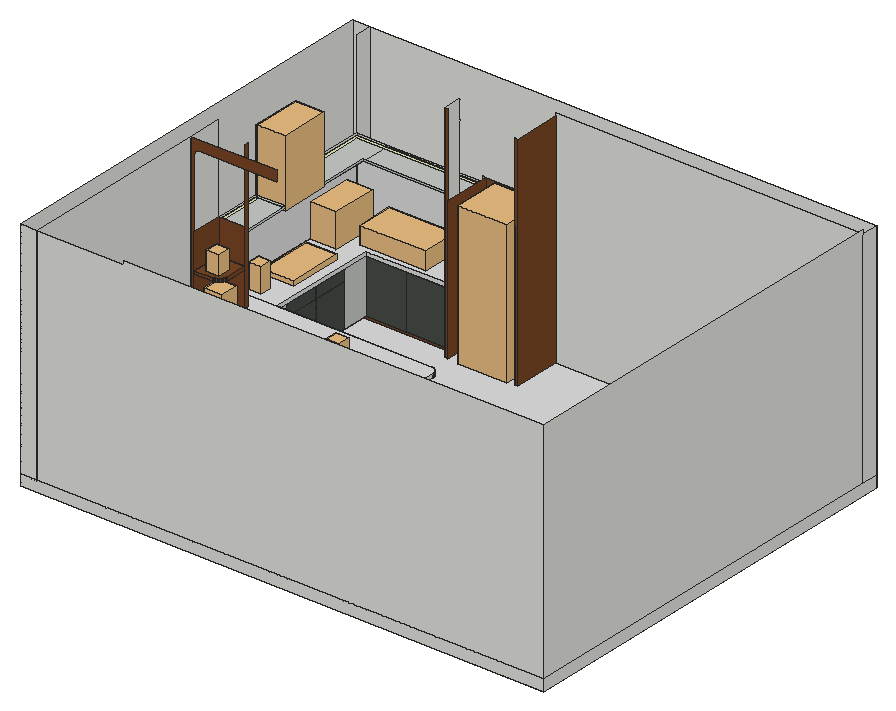
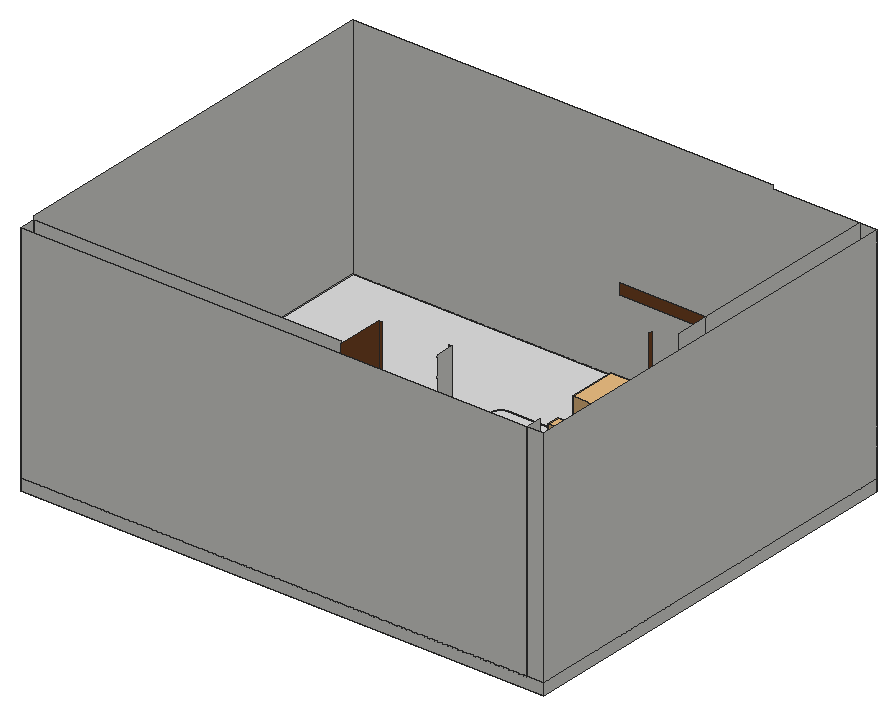
# SketchUp Ruby script. Lengths in inches.
U = 1.inch
M = Sketchup.active_model
def pt(a) = Geom::Point3d.new(a.map { |v| v * U })
def face(e, loops, mat)
  f = e.add_face(loops[0].map { |a| pt(a) })
  loops[1..].each { |l| e.add_face(l.map { |a| pt(a) }).erase! }
  f.material = f.back_material = mat if mat
  f
end
# faces: each face lists its corners as indices into pts; further lists are holes
def faces(e, pts, list, mat = nil) = list.each { |f| face(e, (f[0].is_a?(Array) ? f : [f]).map { |l| l.map { |i| pts[i] } }, mat) }
# xy, xz, yz: faces in a plane at the given z, y or x. An outline is a flat list of corners, or four numbers for a rectangle; further outlines are holes
def ring(l) = l.size == 4 ? [[l[0], l[1]], [l[2], l[1]], [l[2], l[3]], [l[0], l[3]]] : l.each_slice(2).to_a
def flat(e, list, mat, &to3) = list.each { |f| face(e, (f[0].is_a?(Array) ? f : [f]).map { |l| ring(l).map { |u, v| to3.(u, v) } }, mat) }
def xy(e, z, list, mat = nil) = flat(e, list, mat) { |x, y| [x, y, z] }
def xz(e, y, list, mat = nil) = flat(e, list, mat) { |x, z| [x, y, z] }
def yz(e, x, list, mat = nil) = flat(e, list, mat) { |y, z| [x, y, z] }
def lines(e, pts, list) = list.each { |a, b| e.add_line(pt(pts[a]), pt(pts[b])) }
# prism: a flat outline (further loops are holes) pulled along v
def prism(e, loops, v, mat = nil)
  f = face(e, loops, mat); d = Geom::Vector3d.new(v.map { |x| x * U })
  f.pushpull(f.normal.samedirection?(d) ? d.length : -d.length)
end
def box(e, o, s, mat = nil) = prism(e, [[o, [o[0] + s[0], o[1], o[2]], [o[0] + s[0], o[1] + s[1], o[2]], [o[0], o[1] + s[1], o[2]]]], [0, 0, s[2]], mat)
def at(x, y, z, deg = 0) = Geom::Transformation.translation(pt([x, y, z])) * Geom::Transformation.rotation(ORIGIN, Z_AXIS, deg.degrees)
def axes(o, x, y, z) = Geom::Transformation.new([*x, 0, *y, 0, *z, 0, *pt(o).to_a, 1])
def part(name) = M.definitions.add(name)
# library, detail: a bought-in or finely detailed component or shape, given as its bounding box
def library(name, o, s) = part(name).tap { |d| box(d.entities, o, s) }
def detail(e, o, s) = box(e.add_group.entities, o, s)
def put(e, d, t, mat = nil) = e.add_instance(d, t).tap { |i| i.material = mat if mat }
def group(e, t, mat = nil) = e.add_group.tap { |g| g.transformation = t; g.material = mat if mat }.entities
root = M.entities
M.materials.add("Emissive").color = [223, 228, 179]
M.materials.add("Generic").color = [71, 77, 71]
M.materials.add("Generic\#1").color = [198, 203, 199]
M.materials.add("Gold 10k").color = [251, 232, 180]
M.materials.add("Marble White SSS 100cm").color = [222, 222, 222]
M.materials.add("[Wood Veneer 01]").color = [120, 70, 37]
c1 = library("Refrigerator 300 009",[-13.27,-13.92,-0.16],[26.54,24.77,79.78])
c2 = library("Potted Plant 50-23",[-3.4,-3.5,0],[6.8,7,9.93])
c3 = library("Kitchen Sink 180 043",[-17.78,-9.92,-5.26],[35.55,19.84,14.38])
c4 = library("ACCESS \#103",[-1.07,0,-1.17],[14.88,24.44,20.18])
c5 = library("Utensils",[0,-0.54,-0.24],[6.34,6.28,13.37])
c6 = library("GasStove_Black",[0,0,0],[28.74,16.54,2.72])
c7 = library("Vase Lilies 26-19",[-4.61,-5.04,0],[9.42,9.94,10.95])
c8 = library("Tlon Light 1950 Ceiling 152 010",[-38.39,-38.39,-3.78],[76.78,76.78,3.41])
c9 = library("BERG+Spring+90",[0,0,0],[34.65,15.32,35.9])
xy(root,-6,[[0,0,280.625,223.125]])
xy(root,0,[[0,0,9,223.125],[9,0,10.8125,103.125],[9,103.125,10.8125,103.125,10.8125,107.125,33,107.125,33,123.125,29,123.125,29,194.125,33,194.125,33,214.125,9,214.125],[33,107.125,116,123.125],[33,107.125,116,123.125],
  [76.5,188.8125,78.25,188.8125,78.25,214.125,33,214.125,33,194.125,76.5,194.125],[76.5,188.8125,78.25,214.125],[114.125,188.8125,115.875,214.125],[114.125,188.8125,115.875,214.125],[33,194.125,76.5,214.125],
  [9,214.125,280.625,223.125]])
xy(root,0,[[10.8125,0,280.625,0,280.625,214.125,115.875,214.125,115.875,188.8125,114.125,188.8125,114.125,214.125,78.25,214.125,78.25,188.8125,76.5,188.8125,76.5,194.125,29,194.125,29,123.125,116,123.125,116,107.125,10.8125,107.125]],"Marble White SSS 100cm")
xy(root,4,[[10.8125,107.125,10.8125,120.99,9,120.99,9,214.125,76.5,214.125,76.5,194.125,29,194.125,29,123.125,116,123.125,116,107.125]])
xy(root,4,[[10.8125,106.18,10.8125,107.125,116,107.125,116,123.125,29,123.125,29,194.125,76.5,194.125,76.5,193.18,29.95,193.18,29.95,124.07,116.95,124.07,116.95,106.18]],"Emissive")
xy(root,4,[[10.8125,104.5625,10.8125,106.18,21.4375,106.18,21.4375,104.5625,18.3,104.5625,18.3,105.3125,17.9,105.3125,17.9,104.5625,14.75,104.5625,14.75,105.3125,14.35,105.3125,14.35,104.5625],[21.84,104.5625,24.98,106.18],[25.38,104.5625,28.52,106.18],[28.92,104.5625,32.0625,106.18],[99.36,104.5625,99.36,106.18,116.95,106.18,116.95,124.07,29.95,124.07,29.95,193.18,76.5,193.18,76.5,190.125,33,190.125,33,125.6875,117.27,125.6875,117.4375,125.68,117.6,125.64,117.76,125.59,117.92,125.51,118.06,125.42,118.18,125.31,118.29,125.18,118.39,125.04,118.46,124.89,118.52,124.73,118.53,124.6875,118.98,123.14,119.37,121.57,119.68,119.99,119.93,118.39,120.11,116.79,120.21,115.18,120.21,111.95,120.1,110.34,119.92,108.74,119.67,107.14,119.66,107.125,119.35,105.5625,118.48,105.5625,118.45,105.48,118.36,105.31,118.25,105.15,118.125,105,117.98,104.87,117.82,104.76,117.64,104.68,117.46,104.61,117.27,104.58,117.07,104.5625,117.07,105.3125,116.67,105.3125,116.67,104.5625,113.53,104.5625,113.53,105.3125,113.13,105.3125,113.13,104.5625,109.99,104.5625,109.99,105.3125,109.59,105.3125,109.59,104.5625,106.45,104.5625,106.45,105.3125,106.05,105.3125,106.05,104.5625,102.9,104.5625,102.9,105.3125,102.5,105.3125,102.5,104.5625],
  [32.46,104.5625,35.61,106.18],[36.01,104.5625,39.15,106.18],[39.55,104.5625,42.69,106.18],[43.09,104.5625,46.23,106.18],[46.63,104.5625,49.77,106.18],
  [50.17,104.5625,50.17,106.18,91.88,106.18,91.88,104.5625,88.74,104.5625,88.74,105.3125,88.34,105.3125,88.34,104.5625,85.19,104.5625,85.19,105.3125,84.79,105.3125,84.79,104.5625,81.65,104.5625,81.65,105.3125,81.25,105.3125,81.25,104.5625,78.51,104.5625,78.51,105.3125,78.11,105.3125,78.11,104.5625,74.97,104.5625,74.97,105.3125,74.57,105.3125,74.57,104.5625,71.43,104.5625,71.43,105.3125,71.03,105.3125,71.03,104.5625,67.88,104.5625,67.88,105.3125,67.48,105.3125,67.48,104.5625,64.34,104.5625,64.34,105.3125,63.94,105.3125,63.94,104.5625,60.8,104.5625,60.8,105.3125,60.4,105.3125,60.4,104.5625,57.26,104.5625,57.26,105.3125,56.86,105.3125,56.86,104.5625,53.72,104.5625,53.72,105.3125,53.32,105.3125,53.32,104.5625],[92.28,104.5625,95.42,106.18],[95.82,104.5625,98.96,106.18]],"[Wood Veneer 01]")
xy(root,5,[[112.375,105.5625,119.35,105.5625,119.66,107.125,119.67,107.14,119.92,108.74,120.1,110.34,120.21,111.95,120.21,115.18,120.11,116.79,119.93,118.39,119.68,119.99,119.37,121.57,118.98,123.14,118.53,124.6875,112.375,124.6875]],"[Wood Veneer 01]")
xy(root,13.49,[[112.375,105.5625,112.375,124.6875,118.53,124.6875,119.04,123.14,119.47,121.57,119.8,119.98,120.03,118.37,120.17,116.75,120.21,115.12,120.16,113.49,120.01,111.875,119.77,110.26,119.43,108.67,119,107.1,118.48,105.5625]],"[Wood Veneer 01]")
xy(root,14.08,[[112.375,105.5625,118.48,105.5625,119,107.1,119.43,108.67,119.77,110.26,120.01,111.875,120.16,113.49,120.21,115.12,120.17,116.75,120.03,118.37,119.8,119.98,119.47,121.57,119.04,123.14,118.53,124.6875,112.375,124.6875]],"[Wood Veneer 01]")
xy(root,22.24,[[112.375,105.5625,112.375,124.6875,118.53,124.6875,119.04,123.14,119.46,121.57,119.79,119.98,120.03,118.37,120.17,116.75,120.21,115.12,120.16,113.49,120.01,111.875,119.77,110.26,119.43,108.67,119,107.1,118.48,105.5625]],"[Wood Veneer 01]")
xy(root,22.83,[[112.375,105.5625,118.48,105.5625,119,107.1,119.43,108.67,119.77,110.26,120.01,111.875,120.16,113.49,120.21,115.12,120.17,116.75,120.03,118.37,119.79,119.98,119.46,121.57,119.04,123.14,118.53,124.6875,112.375,124.6875]],"[Wood Veneer 01]")
xy(root,32,[[112.375,105.5625,112.375,124.6875,118.53,124.6875,118.55,124.5625,118.5625,124.39,118.5625,106.05,118.55,105.86,118.51,105.67,118.48,105.5625]],"[Wood Veneer 01]")
xy(root,33,[[10.8125,104.5625,10.8125,120.99,9,120.99,9,214.125,76.5,214.125,76.5,190.125,33,190.125,33,125.6875,117.07,125.6875,117.07,105.3125,116.67,105.3125,116.67,104.5625,113.53,104.5625,113.53,105.3125,113.13,105.3125,113.13,104.5625,109.99,104.5625,109.99,105.3125,109.59,105.3125,109.59,104.5625,106.45,104.5625,106.45,105.3125,106.05,105.3125,106.05,104.5625,102.9,104.5625,102.9,105.3125,102.5,105.3125,102.5,104.5625,99.36,104.5625,99.36,106.18,98.96,106.18,98.96,104.5625,95.82,104.5625,95.82,106.18,95.42,106.18,95.42,104.5625,92.28,104.5625,92.28,106.18,91.88,106.18,91.88,104.5625,88.74,104.5625,88.74,105.3125,88.34,105.3125,88.34,104.5625,85.19,104.5625,85.19,105.3125,84.79,105.3125,84.79,104.5625,81.65,104.5625,81.65,105.3125,81.25,105.3125,81.25,104.5625,78.51,104.5625,78.51,105.3125,78.11,105.3125,78.11,104.5625,74.97,104.5625,74.97,105.3125,74.57,105.3125,74.57,104.5625,71.43,104.5625,71.43,105.3125,71.03,105.3125,71.03,104.5625,67.88,104.5625,67.88,105.3125,67.48,105.3125,67.48,104.5625,64.34,104.5625,64.34,105.3125,63.94,105.3125,63.94,104.5625,60.8,104.5625,60.8,105.3125,60.4,105.3125,60.4,104.5625,57.26,104.5625,57.26,105.3125,56.86,105.3125,56.86,104.5625,53.72,104.5625,53.72,105.3125,53.32,105.3125,53.32,104.5625,50.17,104.5625,50.17,106.18,49.77,106.18,49.77,104.5625,46.63,104.5625,46.63,106.18,46.23,106.18,46.23,104.5625,43.09,104.5625,43.09,106.18,42.69,106.18,42.69,104.5625,39.55,104.5625,39.55,106.18,39.15,106.18,39.15,104.5625,36.01,104.5625,36.01,106.18,35.61,106.18,35.61,104.5625,32.46,104.5625,32.46,106.18,32.0625,106.18,32.0625,104.5625,28.92,104.5625,28.92,106.18,28.52,106.18,28.52,104.5625,25.38,104.5625,25.38,106.18,24.98,106.18,24.98,104.5625,21.84,104.5625,21.84,106.18,21.4375,106.18,21.4375,104.5625,18.3,104.5625,18.3,105.3125,17.9,105.3125,17.9,104.5625,14.75,104.5625,14.75,105.3125,14.35,105.3125,14.35,104.5625],[117.07,104.5625,117.27,104.58,117.46,104.61,117.64,104.68,117.82,104.76,117.98,104.87,118.125,105,118.25,105.15,118.36,105.31,118.45,105.48,118.51,105.67,118.55,105.86,118.5625,106.05,118.5625,124.39,118.55,124.5625,118.52,124.73,118.46,124.89,118.39,125.04,118.29,125.18,118.18,125.31,118.06,125.42,117.92,125.51,117.76,125.59,117.6,125.64,117.4375,125.68,117.27,125.6875,117.07,125.6875]])
xy(root,33,[[10.8125,103.8125,10.8125,104.5625,14.35,104.5625,14.35,105.3125,14.75,105.3125,14.75,104.5625,17.9,104.5625,17.9,105.3125,18.3,105.3125,18.3,104.5625,21.4375,104.5625,21.4375,106.18,21.84,106.18,21.84,104.5625,24.98,104.5625,24.98,106.18,25.38,106.18,25.38,104.5625,28.52,104.5625,28.52,106.18,28.92,106.18,28.92,104.5625,32.0625,104.5625,32.0625,106.18,32.46,106.18,32.46,104.5625,35.61,104.5625,35.61,106.18,36.01,106.18,36.01,104.5625,39.15,104.5625,39.15,106.18,39.55,106.18,39.55,104.5625,42.69,104.5625,42.69,106.18,43.09,106.18,43.09,104.5625,46.23,104.5625,46.23,106.18,46.63,106.18,46.63,104.5625,49.77,104.5625,49.77,106.18,50.17,106.18,50.17,104.5625,53.32,104.5625,53.32,105.3125,53.72,105.3125,53.72,104.5625,56.86,104.5625,56.86,105.3125,57.26,105.3125,57.26,104.5625,60.4,104.5625,60.4,105.3125,60.8,105.3125,60.8,104.5625,63.94,104.5625,63.94,105.3125,64.34,105.3125,64.34,104.5625,67.48,104.5625,67.48,105.3125,67.88,105.3125,67.88,104.5625,71.03,104.5625,71.03,105.3125,71.43,105.3125,71.43,104.5625,74.57,104.5625,74.57,105.3125,74.97,105.3125,74.97,104.5625,78.11,104.5625,78.11,105.3125,78.51,105.3125,78.51,104.5625,81.25,104.5625,81.25,105.3125,81.65,105.3125,81.65,104.5625,84.79,104.5625,84.79,105.3125,85.19,105.3125,85.19,104.5625,88.34,104.5625,88.34,105.3125,88.74,105.3125,88.74,104.5625,91.88,104.5625,91.88,106.18,92.28,106.18,92.28,104.5625,95.42,104.5625,95.42,106.18,95.82,106.18,95.82,104.5625,98.96,104.5625,98.96,106.18,99.36,106.18,99.36,104.5625,102.5,104.5625,102.5,105.3125,102.9,105.3125,102.9,104.5625,106.05,104.5625,106.05,105.3125,106.45,105.3125,106.45,104.5625,109.59,104.5625,109.59,105.3125,109.99,105.3125,109.99,104.5625,113.13,104.5625,113.13,105.3125,113.53,105.3125,113.53,104.5625,116.67,104.5625,116.67,105.3125,117.07,105.3125,117.07,103.8125],[117.07,103.8125,117.07,104.5625,117.27,104.58,117.46,104.61,117.64,104.68,117.82,104.76,117.98,104.87,118.125,105,118.25,105.15,118.36,105.31,118.45,105.48,118.51,105.67,118.55,105.86,118.5625,106.05,118.5625,124.39,118.55,124.5625,118.52,124.73,118.46,124.89,118.39,125.04,118.29,125.18,118.18,125.31,118.06,125.42,117.92,125.51,117.76,125.59,117.6,125.64,117.4375,125.68,117.27,125.6875,117.07,125.6875,117.07,126.4375,119.125,126.4375,119.125,103.8125],[33,125.6875,117.07,126.4375]],"Emissive")
xy(root,34,[[120.76,103.125,120.8125,103.125,120.8125,103.21],[120.8125,103.21,120.99,103.48,121.27,104.03,121.46,104.62,121.58,105.22,121.625,105.83,121.625,124.4,121.58,125.02,121.46,125.62,121.27,126.21,120.99,126.76,120.8125,127.03],[10.8125,103.8125,10.8125,120.99,9,120.99,9,214.125,76.5,214.125,76.5,190.125,33,190.125,33,126.4375,117.07,126.4375,117.07,103.8125],[120.8125,127.03,120.8125,127.125,120.75,127.125]])
xy(root,34,[[10.8125,101.125,10.8125,103.8125,119.9375,103.8125,119.9375,103.125,120.76,103.125,120.65,102.97,120.25,102.5,119.78,102.1,119.27,101.76,118.72,101.48,118.13,101.29,117.53,101.17,116.92,101.125],[119.9375,103.125,120.76,103.125,120.8125,103.21,120.8125,127.03,120.75,127.125,119.9375,127.125,119.9375,126.4375,119.125,126.4375,119.125,103.8125,119.9375,103.8125],[33,126.4375,33,129.125,116.9,129.125,117.52,129.08,118.12,128.96,118.71,128.77,119.26,128.49,119.78,128.15,120.24,127.74,120.65,127.28,120.75,127.125,119.9375,127.125,119.9375,126.4375],[33,129.125,34.3125,188.8125],[33,188.8125,76.5,190.125]],"Marble White SSS 100cm")
xy(root,36,[[10.8125,119.26,25,120.99]])
xy(root,36,[[10.8125,101.125,116.92,101.125,117.53,101.17,118.13,101.29,118.72,101.48,119.27,101.76,119.78,102.1,120.25,102.5,120.65,102.97,120.99,103.48,121.27,104.03,121.46,104.62,121.58,105.22,121.625,105.83,121.625,124.4,121.58,125.02,121.46,125.62,121.27,126.21,120.99,126.76,120.65,127.28,120.24,127.74,119.78,128.15,119.26,128.49,118.71,128.77,118.12,128.96,117.52,129.08,116.9,129.125,9,129.125,9,120.99,25,120.99,25,119.26,10.8125,119.26],[9,129.125,34.3125,129.125,34.3125,188.8125,76.5,188.8125,76.5,214.125,9,214.125]],"Marble White SSS 100cm")
xy(root,54.52,[[10.8125,103.125,10.8125,119.26,25,119.26,25,107.5625,24.96,106.98,24.85,106.41,24.66,105.86,24.41,105.34,24.08,104.86,23.7,104.42,23.26,104.04,22.78,103.72,22.26,103.46,21.71,103.28,21.14,103.16,20.5625,103.125]],"[Wood Veneer 01]")
xy(root,56.22,[[10.8125,103.125,20.5625,103.125,21.14,103.16,21.71,103.28,22.26,103.46,22.78,103.72,23.26,104.04,23.7,104.42,24.08,104.86,24.41,105.34,24.66,105.86,24.85,106.41,24.96,106.98,25,107.5625,25,119.26,10.8125,119.26]],"[Wood Veneer 01]")
xy(root,72,[[9,120.99,11,146.7],[9,172.41,9,214.125,76.5,214.125,76.5,212.125,11,212.125,11,172.41]],"Emissive")
xy(root,72,[[11,120.99,25,146.7],[11,172.41,25,212.125],[25,198.125,76.5,212.125]],"Generic\#1")
xz(root,0,[[0,-6,280.625,0],[0,0,9,120],[9,0,280.625,0,280.625,122,55.3125,122,55.3125,120,9,120]])
xz(root,101.125,[[10.8125,34,116.92,36]])
xz(root,103.125,[[9,0,10.8125,0,10.8125,112.09,10.83,112.4,10.89,112.71,10.99,113,11.13,113.29,11.31,113.55,11.51,113.78,11.75,113.99,12.01,114.16,12.29,114.3,12.59,114.4,12.89,114.46,13.21,114.48,55.3125,114.48,55.3125,120,9,120],[10.8125,54.52,20.5625,56.22]],"[Wood Veneer 01]")
xz(root,103.8125,[[10.8125,33,117.07,34],[117.07,33,119.125,34]],"[Wood Veneer 01]")
xz(root,104.5625,[[10.8125,4,14.35,33],[14.75,4,17.9,33],[18.3,4,21.4375,33],[21.84,4,24.98,33],[25.38,4,28.52,33],
  [28.92,4,32.0625,33],[32.46,4,35.61,33],[36.01,4,39.15,33],[39.55,4,42.69,33],[43.09,4,46.23,33],
  [46.63,4,49.77,33],[50.17,4,53.32,33],[53.72,4,56.86,33],[57.26,4,60.4,33],[60.8,4,63.94,33],
  [64.34,4,67.48,33],[67.88,4,71.03,33],[71.43,4,74.57,33],[74.97,4,78.11,33],[78.51,4,81.25,33],
  [81.65,4,84.79,33],[85.19,4,88.34,33],[88.74,4,91.88,33],[92.28,4,95.42,33],[95.82,4,98.96,33],
  [99.36,4,102.5,33],[102.9,4,106.05,33],[106.45,4,109.59,33],[109.99,4,113.13,33],[113.53,4,116.67,33]],"Generic")
xz(root,105.3125,[[14.35,4,14.75,33],[17.9,4,18.3,33],[53.32,4,53.72,33],[56.86,4,57.26,33],[60.4,4,60.8,33],
  [63.94,4,64.34,33],[67.48,4,67.88,33],[71.03,4,71.43,33],[74.57,4,74.97,33],[78.11,4,78.51,33],
  [81.25,4,81.65,33],[84.79,4,85.19,33],[88.34,4,88.74,33],[102.5,4,102.9,33],[106.05,4,106.45,33],
  [109.59,4,109.99,33],[113.13,4,113.53,33],[116.67,4,117.07,33]],"Gold 10k")
xz(root,105.5625,[[118.48,4,119.35,5],[112.375,5,118.48,13.49],[112.375,14.08,118.48,22.24],[112.375,22.83,118.48,32]],"[Wood Veneer 01]")
xz(root,106.18,[[21.4375,4,21.84,33],[24.98,4,25.38,33],[28.52,4,28.92,33],[32.0625,4,32.46,33],[35.61,4,36.01,33],
  [39.15,4,39.55,33],[42.69,4,43.09,33],[46.23,4,46.63,33],[49.77,4,50.17,33],[91.88,4,92.28,33],
  [95.42,4,95.82,33],[98.96,4,99.36,33]],"Gold 10k")
xz(root,107.125,[[10.8125,0,116,4]],"[Wood Veneer 01]")
xz(root,119.26,[[10.8125,54.52,25,56.22]])
xz(root,119.26,[[10.8125,36,25,54.52],[10.8125,56.22,25,75.04]],"[Wood Veneer 01]")
xz(root,120.99,[[9,4,10.8125,33],[9,33,10.8125,34],[9,34,10.8125,36],[9,72,25,72.9375]])
xz(root,120.99,[[9,36,25,72]],"Marble White SSS 100cm")
xz(root,123.125,[[29,0,116,4]],"[Wood Veneer 01]")
xz(root,124.6875,[[112.375,5,118.53,13.49],[112.375,14.08,118.53,22.24],[112.375,22.83,118.53,32]],"[Wood Veneer 01]")
xz(root,125.6875,[[33,4,117.27,33]],"Generic")
xz(root,126.4375,[[33,33,117.07,34],[117.07,33,119.125,34]],"Generic")
xz(root,129.125,[[34.3125,34,116.9,36]])
xz(root,146.7,[[9,72,25,72.9375]])
xz(root,172.41,[[9,72,25,72.9375]],"Generic\#1")
xz(root,188.8125,[[34.3125,34,76.5,36]],"Marble White SSS 100cm")
xz(root,188.8125,[[76.5,0,78.25,120],[114.125,0,115.875,118.5]],"[Wood Veneer 01]")
xz(root,190.125,[[33,33,76.5,34]])
xz(root,190.125,[[33,4,54.75,33],[55.15,4,76.5,33]],"Generic")
xz(root,190.125,[[54.75,4,55.15,33]],"Gold 10k")
xz(root,194.125,[[29,0,76.5,4]],"[Wood Veneer 01]")
xz(root,198.125,[[25,72,76.5,72.9375]],"Generic\#1")
xz(root,214.125,[[9,0,33,4],[33,0,76.5,4],[76.5,0,78.25,75.875],[114.125,0,115.875,75.875],[115.875,0,280.625,120],
  [9,4,33,33],[33,4,76.5,33],[9,33,33,34],[33,33,76.5,34],[9,34,33,36],
  [33,34,76.5,36],[9,72,25,72.9375],[25,72,76.5,72.9375]])
xz(root,214.125,[[9,36,76.5,72]],"Marble White SSS 100cm")
xz(root,214.125,[[78.25,0,114.125,75.875]],"[Wood Veneer 01]")
xz(root,223.125,[[0,-6,280.625,0],[0,0,9,120],[9,0,280.625,120]])
yz(root,0,[[0,-6,223.125,0],[0,0,223.125,120]])
yz(root,9,[[0,0,103.125,36],[103.125,0,103.125,36,120.99,36,120.99,4,214.125,4,214.125,0],[214.125,0,223.125,120],[120.99,4,214.125,33],[120.99,33,214.125,34],
  [120.99,34,214.125,36],[0,36,103.125,120],[103.125,36,120.99,120],[120.99,72,146.7,72.9375],[172.41,72,214.125,72.9375]])
yz(root,9,[[120.99,36,214.125,36,214.125,72,172.41,72,172.41,106.4375,146.7,106.4375,146.7,72,120.99,72]],"Marble White SSS 100cm")
yz(root,10.8125,[[104.5625,4,120.99,33],[103.8125,33,120.99,34],[101.125,34,103.125,36],[103.125,34,120.99,36],[103.125,54.52,119.26,56.22]])
yz(root,10.8125,[[103.125,0,107.125,4]],"Generic")
yz(root,10.8125,[[103.125,4,104.5625,33],[103.125,33,103.8125,34],[103.125,36,119.26,54.52],[103.125,56.22,119.26,75.04]],"[Wood Veneer 01]")
yz(root,14.35,[[104.5625,4,105.3125,33]],"Gold 10k")
yz(root,14.75,[[104.5625,4,105.3125,33]],"Gold 10k")
yz(root,17.9,[[104.5625,4,105.3125,33]],"Gold 10k")
yz(root,18.3,[[104.5625,4,105.3125,33]],"Gold 10k")
yz(root,21.4375,[[104.5625,4,106.18,33]],"Gold 10k")
yz(root,21.84,[[104.5625,4,106.18,33]],"Gold 10k")
yz(root,24.98,[[104.5625,4,106.18,33]],"Gold 10k")
yz(root,25,[[120.99,72,146.7,72.9375],[172.41,72,198.125,72.9375]],"Generic\#1")
yz(root,25,[[119.26,36,120.99,114.48],[107.5625,54.52,119.26,56.22]],"[Wood Veneer 01]")
yz(root,25.38,[[104.5625,4,106.18,33]],"Gold 10k")
yz(root,28.52,[[104.5625,4,106.18,33]],"Gold 10k")
yz(root,28.92,[[104.5625,4,106.18,33]],"Gold 10k")
yz(root,29,[[123.125,0,194.125,4]],"[Wood Veneer 01]")
yz(root,32.0625,[[104.5625,4,106.18,33]],"Gold 10k")
yz(root,32.46,[[104.5625,4,106.18,33]],"Gold 10k")
yz(root,33,[[126.4375,33,190.125,34]])
yz(root,33,[[137.47,4,156.55,26.45],[156.95,4,176.03,26.45],[137.47,26.85,156.55,33],[156.95,26.85,176.03,33]],"Generic")
yz(root,33,[[125.6875,4,137.07,33],[176.43,4,190.125,33]],"Generic\#1")
yz(root,33,[[137.07,4,137.47,33],[156.55,4,156.95,33],[176.03,4,176.43,33],[137.47,26.45,156.55,26.85],[156.95,26.45,176.03,26.85]],"Gold 10k")
yz(root,34.3125,[[129.125,34,188.8125,36]],"Marble White SSS 100cm")
yz(root,35.61,[[104.5625,4,106.18,33]],"Gold 10k")
yz(root,36.01,[[104.5625,4,106.18,33]],"Gold 10k")
yz(root,39.15,[[104.5625,4,106.18,33]],"Gold 10k")
yz(root,39.55,[[104.5625,4,106.18,33]],"Gold 10k")
yz(root,42.69,[[104.5625,4,106.18,33]],"Gold 10k")
yz(root,43.09,[[104.5625,4,106.18,33]],"Gold 10k")
yz(root,46.23,[[104.5625,4,106.18,33]],"Gold 10k")
yz(root,46.63,[[104.5625,4,106.18,33]],"Gold 10k")
yz(root,49.77,[[104.5625,4,106.18,33]],"Gold 10k")
yz(root,50.17,[[104.5625,4,106.18,33]],"Gold 10k")
yz(root,53.32,[[104.5625,4,105.3125,33]],"Gold 10k")
yz(root,53.72,[[104.5625,4,105.3125,33]],"Gold 10k")
yz(root,56.86,[[104.5625,4,105.3125,33]],"Gold 10k")
yz(root,57.26,[[104.5625,4,105.3125,33]],"Gold 10k")
yz(root,60.4,[[104.5625,4,105.3125,33]],"Gold 10k")
yz(root,60.8,[[104.5625,4,105.3125,33]],"Gold 10k")
yz(root,63.94,[[104.5625,4,105.3125,33]],"Gold 10k")
yz(root,64.34,[[104.5625,4,105.3125,33]],"Gold 10k")
yz(root,67.48,[[104.5625,4,105.3125,33]],"Gold 10k")
yz(root,67.88,[[104.5625,4,105.3125,33]],"Gold 10k")
yz(root,71.03,[[104.5625,4,105.3125,33]],"Gold 10k")
yz(root,71.43,[[104.5625,4,105.3125,33]],"Gold 10k")
yz(root,74.57,[[104.5625,4,105.3125,33]],"Gold 10k")
yz(root,74.97,[[104.5625,4,105.3125,33]],"Gold 10k")
yz(root,76.5,[[188.8125,0,188.8125,34,190.125,34,190.125,4,194.125,4,194.125,0],[194.125,0,214.125,4],[190.125,4,214.125,33],[190.125,33,214.125,34],[188.8125,34,214.125,36],
  [188.8125,36,188.8125,120,198.125,120,198.125,119.4375,198.875,119.4375,198.875,119.1875,198.125,119.1875,198.125,109.43,198.875,109.43,198.875,109.03,198.125,109.03,198.125,73.34,198.875,73.34,198.875,72.9375,198.125,72.9375,198.125,72,214.125,72,214.125,36],[198.125,72,214.125,72.9375]])
yz(root,78.11,[[104.5625,4,105.3125,33]],"Gold 10k")
yz(root,78.25,[[188.8125,0,214.125,75.875]],"[Wood Veneer 01]")
yz(root,78.51,[[104.5625,4,105.3125,33]],"Gold 10k")
yz(root,81.25,[[104.5625,4,105.3125,33]],"Gold 10k")
yz(root,81.65,[[104.5625,4,105.3125,33]],"Gold 10k")
yz(root,84.79,[[104.5625,4,105.3125,33]],"Gold 10k")
yz(root,85.19,[[104.5625,4,105.3125,33]],"Gold 10k")
yz(root,88.34,[[104.5625,4,105.3125,33]],"Gold 10k")
yz(root,88.74,[[104.5625,4,105.3125,33]],"Gold 10k")
yz(root,91.88,[[104.5625,4,106.18,33]],"Gold 10k")
yz(root,92.28,[[104.5625,4,106.18,33]],"Gold 10k")
yz(root,95.42,[[104.5625,4,106.18,33]],"Gold 10k")
yz(root,95.82,[[104.5625,4,106.18,33]],"Gold 10k")
yz(root,98.96,[[104.5625,4,106.18,33]],"Gold 10k")
yz(root,99.36,[[104.5625,4,106.18,33]],"Gold 10k")
yz(root,102.5,[[104.5625,4,105.3125,33]],"Gold 10k")
yz(root,102.9,[[104.5625,4,105.3125,33]],"Gold 10k")
yz(root,106.05,[[104.5625,4,105.3125,33]],"Gold 10k")
yz(root,106.45,[[104.5625,4,105.3125,33]],"Gold 10k")
yz(root,109.59,[[104.5625,4,105.3125,33]],"Gold 10k")
yz(root,109.99,[[104.5625,4,105.3125,33]],"Gold 10k")
yz(root,112.375,[[105.5625,5,124.6875,13.49],[105.5625,14.08,124.6875,22.24],[105.5625,22.83,124.6875,32]],"[Wood Veneer 01]")
yz(root,113.13,[[104.5625,4,105.3125,33]],"Gold 10k")
yz(root,113.53,[[104.5625,4,105.3125,33]],"Gold 10k")
yz(root,114.125,[[188.8125,0,214.125,75.875]],"[Wood Veneer 01]")
yz(root,115.875,[[188.8125,0,214.125,118.5]],"[Wood Veneer 01]")
yz(root,116,[[107.125,0,123.125,4]],"[Wood Veneer 01]")
yz(root,116.67,[[104.5625,4,105.3125,33]],"Gold 10k")
yz(root,117.07,[[103.8125,33,126.4375,34]])
yz(root,117.07,[[104.5625,4,105.3125,33]],"Gold 10k")
yz(root,118.5625,[[106.05,32,124.39,33]],"[Wood Veneer 01]")
yz(root,119.125,[[103.8125,33,126.4375,34]],"[Wood Veneer 01]")
yz(root,120.21,[[111.95,4,112.25,5],[112.25,4,115.07,5],[115.07,4,115.18,5]],"[Wood Veneer 01]")
yz(root,121.625,[[105.83,34,124.4,36]],"Marble White SSS 100cm")
yz(root,280.625,[[0,-6,223.125,0],[0,0,214.125,122],[214.125,0,223.125,120]])
p = [[117.07,104.5625,33],[117.27,104.58,33],[117.27,104.58,4],[117.07,104.5625,4],[117.46,104.61,33],[117.46,104.61,4],
  [117.64,104.68,33],[117.64,104.68,4],[117.82,104.76,33],[117.82,104.76,4],[117.98,104.87,33],[117.98,104.87,4],
  [118.125,105,33],[118.125,105,4],[118.25,105.15,33],[118.25,105.15,4],[118.36,105.31,33],[118.36,105.31,4],
  [118.45,105.48,33],[118.45,105.48,4],[118.51,105.67,33],[118.51,105.67,32],[118.48,105.5625,32],[118.48,105.5625,22.83],
  [118.48,105.5625,22.24],[118.48,105.5625,14.08],[118.48,105.5625,13.49],[118.48,105.5625,5],[118.48,105.5625,4],[119.66,107.125,5],
  [119.35,105.5625,5],[119.35,105.5625,4],[119.66,107.125,4],[119.92,108.74,5],[119.67,107.14,5],[119.67,107.14,4],
  [119.92,108.74,4],[120.1,110.34,5],[120.1,110.34,4],[120.21,111.95,5],[120.21,111.95,4],[120.11,116.79,5],
  [120.21,115.18,5],[120.21,115.18,4],[120.11,116.79,4],[119.93,118.39,5],[119.93,118.39,4],[119.68,119.99,5],
  [119.68,119.99,4],[119.37,121.57,5],[119.37,121.57,4],[118.98,123.14,5],[118.98,123.14,4],[118.53,124.6875,5],
  [118.53,124.6875,4],[118.55,124.5625,33],[118.52,124.73,33],[118.52,124.73,4],[118.53,124.6875,13.49],[118.53,124.6875,14.08],
  [118.53,124.6875,22.24],[118.53,124.6875,22.83],[118.53,124.6875,32],[118.55,124.5625,32],[118.46,124.89,33],[118.46,124.89,4],
  [118.39,125.04,33],[118.39,125.04,4],[118.29,125.18,33],[118.29,125.18,4],[118.18,125.31,33],[118.18,125.31,4],
  [118.06,125.42,33],[118.06,125.42,4],[117.92,125.51,33],[117.92,125.51,4],[117.76,125.59,33],[117.76,125.59,4],
  [117.6,125.64,33],[117.4375,125.68,33],[117.4375,125.68,4],[117.6,125.64,4],[117.27,125.6875,33],[117.27,125.6875,4],
  [119,107.1,14.08],[119,107.1,13.49],[119.43,108.67,14.08],[119.43,108.67,13.49],[119.77,110.26,14.08],[119.77,110.26,13.49],
  [120.01,111.875,14.08],[120.01,111.875,13.49],[120.16,113.49,14.08],[120.16,113.49,13.49],[120.21,115.12,14.08],[120.21,115.12,13.49],
  [120.17,116.75,14.08],[120.17,116.75,13.49],[120.03,118.37,14.08],[120.03,118.37,13.49],[119.8,119.98,14.08],[119.8,119.98,13.49],
  [119.47,121.57,14.08],[119.47,121.57,13.49],[119.04,123.14,14.08],[119.04,123.14,13.49],[119,107.1,22.83],[119,107.1,22.24],
  [119.43,108.67,22.83],[119.43,108.67,22.24],[119.77,110.26,22.83],[119.77,110.26,22.24],[120.01,111.875,22.83],[120.01,111.875,22.24],
  [120.16,113.49,22.83],[120.16,113.49,22.24],[120.21,115.12,22.83],[120.21,115.12,22.24],[120.17,116.75,22.83],[120.17,116.75,22.24],
  [120.03,118.37,22.83],[120.03,118.37,22.24],[119.79,119.98,22.83],[119.79,119.98,22.24],[119.46,121.57,22.83],[119.46,121.57,22.24],
  [119.04,123.14,22.83],[119.04,123.14,22.24],[118.55,105.86,33],[118.55,105.86,32],[118.5625,106.05,33],[118.5625,106.05,32],
  [118.5625,124.39,33],[118.5625,124.39,32],[117.53,101.17,36],[116.92,101.125,36],[116.92,101.125,34],[117.53,101.17,34],
  [118.13,101.29,36],[118.13,101.29,34],[118.72,101.48,36],[118.72,101.48,34],[119.27,101.76,36],[119.27,101.76,34],
  [119.78,102.1,36],[119.78,102.1,34],[120.25,102.5,36],[120.25,102.5,34],[120.65,102.97,36],[120.65,102.97,34],
  [120.99,103.48,36],[120.76,103.125,34],[120.8125,103.21,34],[120.99,103.48,34],[121.27,104.03,36],[121.27,104.03,34],
  [121.46,104.62,36],[121.46,104.62,34],[121.58,105.22,36],[121.58,105.22,34],[121.625,105.83,36],[121.625,105.83,34],
  [121.58,125.02,36],[121.625,124.4,36],[121.625,124.4,34],[121.58,125.02,34],[121.46,125.62,36],[121.46,125.62,34],
  [121.27,126.21,36],[121.27,126.21,34],[120.99,126.76,36],[120.99,126.76,34],[120.65,127.28,36],[120.8125,127.03,34],
  [120.75,127.125,34],[120.65,127.28,34],[120.24,127.74,36],[120.24,127.74,34],[119.78,128.15,36],[119.78,128.15,34],
  [119.26,128.49,36],[119.26,128.49,34],[118.71,128.77,36],[118.71,128.77,34],[118.12,128.96,36],[118.12,128.96,34],
  [117.52,129.08,36],[117.52,129.08,34],[116.9,129.125,36],[116.9,129.125,34],[21.14,103.16,56.22],[20.5625,103.125,56.22],
  [20.5625,103.125,54.52],[21.14,103.16,54.52],[21.71,103.28,56.22],[21.71,103.28,54.52],[22.26,103.46,56.22],[22.26,103.46,54.52],
  [22.78,103.72,56.22],[22.78,103.72,54.52],[23.26,104.04,56.22],[23.26,104.04,54.52],[23.7,104.42,56.22],[23.7,104.42,54.52],
  [24.08,104.86,56.22],[24.08,104.86,54.52],[24.41,105.34,56.22],[24.41,105.34,54.52],[24.66,105.86,56.22],[24.66,105.86,54.52],
  [24.85,106.41,56.22],[24.85,106.41,54.52],[24.96,106.98,56.22],[24.96,106.98,54.52],[25,107.5625,56.22],[25,107.5625,54.52],
  [10.8125,106.18,4],[10.32,106.18,4],[32.05,156.95,4],[32.05,156.55,4],[32.05,137.47,4],[32.05,137.07,4]]
faces(root,p,[[0,1,2,3],[1,4,5,2],[4,6,7,5],[6,8,9,7],[8,10,11,9],[10,12,13,11],[12,14,15,13],[14,16,17,15],
  [16,18,19,17],[18,20,21,22,23,24,25,26,27,28,19],[29,30,31,32],[33,34,35,36],[34,29,32,35],[37,33,36,38],[39,37,38,40],[41,42,43,44],
  [45,41,44,46],[47,45,46,48],[49,47,48,50],[51,49,50,52],[53,51,52,54],[55,56,57,54,53,58,59,60,61,62,63],[56,64,65,57],[64,66,67,65],
  [66,68,69,67],[68,70,71,69],[70,72,73,71],[72,74,75,73],[74,76,77,75],[78,79,80,81],[76,78,81,77],[79,82,83,80],
  [84,25,26,85],[86,84,85,87],[88,86,87,89],[90,88,89,91],[92,90,91,93],[94,92,93,95],[96,94,95,97],[98,96,97,99],
  [100,98,99,101],[102,100,101,103],[104,102,103,105],[59,104,105,58],[106,23,24,107],[108,106,107,109],[110,108,109,111],[112,110,111,113],
  [114,112,113,115],[116,114,115,117],[118,116,117,119],[120,118,119,121],[122,120,121,123],[124,122,123,125],[126,124,125,127],[61,126,127,60],
  [20,128,129,21],[128,130,131,129],[132,55,63,133],[190,191,192,193],[194,190,193,195],[196,194,195,197],[198,196,197,199],[200,198,199,201],
  [202,200,201,203],[204,202,203,205],[206,204,205,207],[208,206,207,209],[210,208,209,211],[212,210,211,213],[214,212,213,215]],"[Wood Veneer 01]")
faces(root,p,[[134,135,136,137],[138,134,137,139],[140,138,139,141],[142,140,141,143],[144,142,143,145],[146,144,145,147],[148,146,147,149],[150,148,149,151,152,153],
  [154,150,153,155],[156,154,155,157],[158,156,157,159],[160,158,159,161],[162,163,164,165],[166,162,165,167],[168,166,167,169],[170,168,169,171],
  [172,170,171,173,174,175],[176,172,175,177],[178,176,177,179],[180,178,179,181],[182,180,181,183],[184,182,183,185],[186,184,185,187],[188,186,187,189]],"Marble White SSS 100cm")
lines(root,p,[[216,217],[218,219],[219,220],[220,221]])
put(root,c1,axes([97.21,202.06,-0.01],[1,0,0],[0,1,0],[0,0,0.95305]))
put(root,c2,axes([116.61,113.2,5],[1.005,0,0],[0,1.08,0],[0,0,0.75]))
put(root,c2,axes([115.67,113.8,22.83],[1.1968,0,0],[0,1.2672,0],[0,0,0.88]))
put(root,c3,at(46.19,201.83,36))
put(root,c4,at(9.42,182.8125,34.75))
put(root,c5,at(16.15,133.71,36))
put(root,c6,at(29.16,146.91,35.88,90))
put(root,c7,at(17.82,111.85,36))
put(root,c2,at(82.375,109.6,36))
put(root,c8,axes([16.31,114.24,54.61],[0.0252,0,0],[0,0.0252,0],[0,0,0.0252]))
put(root,c2,at(18.23,109.55,56.22))
put(root,c9,axes([25,146.7,70.91],[0,0.74208,0],[-1,0,0],[0,0,1]))
